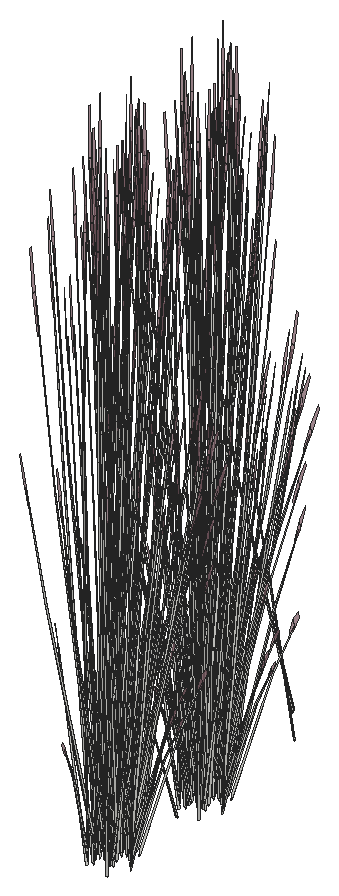
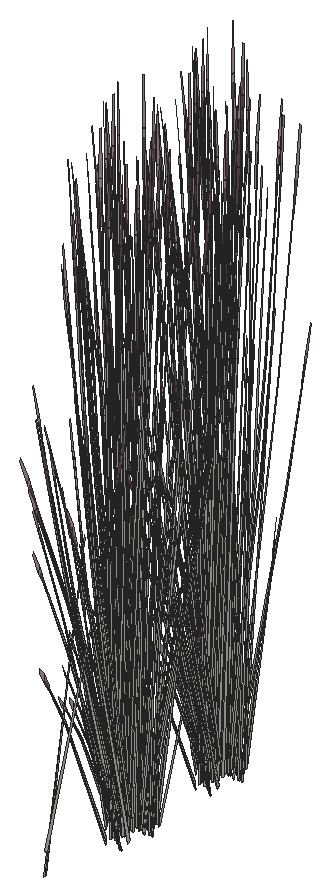
# SketchUp Ruby script. Lengths in inches.
U = 1.inch
M = Sketchup.active_model
def pt(a) = Geom::Point3d.new(a.map { |v| v * U })
def face(e, loops, mat)
  f = e.add_face(loops[0].map { |a| pt(a) })
  loops[1..].each { |l| e.add_face(l.map { |a| pt(a) }).erase! }
  f.material = f.back_material = mat if mat
  f
end
# faces: each face lists its corners as indices into pts; further lists are holes
def faces(e, pts, list, mat = nil) = list.each { |f| face(e, (f[0].is_a?(Array) ? f : [f]).map { |l| l.map { |i| pts[i] } }, mat) }
# xy, xz, yz: faces in a plane at the given z, y or x. An outline is a flat list of corners, or four numbers for a rectangle; further outlines are holes
def ring(l) = l.size == 4 ? [[l[0], l[1]], [l[2], l[1]], [l[2], l[3]], [l[0], l[3]]] : l.each_slice(2).to_a
def flat(e, list, mat, &to3) = list.each { |f| face(e, (f[0].is_a?(Array) ? f : [f]).map { |l| ring(l).map { |u, v| to3.(u, v) } }, mat) }
def xy(e, z, list, mat = nil) = flat(e, list, mat) { |x, y| [x, y, z] }
def xz(e, y, list, mat = nil) = flat(e, list, mat) { |x, z| [x, y, z] }
def yz(e, x, list, mat = nil) = flat(e, list, mat) { |y, z| [x, y, z] }
def lines(e, pts, list) = list.each { |a, b| e.add_line(pt(pts[a]), pt(pts[b])) }
# prism: a flat outline (further loops are holes) pulled along v
def prism(e, loops, v, mat = nil)
  f = face(e, loops, mat); d = Geom::Vector3d.new(v.map { |x| x * U })
  f.pushpull(f.normal.samedirection?(d) ? d.length : -d.length)
end
def box(e, o, s, mat = nil) = prism(e, [[o, [o[0] + s[0], o[1], o[2]], [o[0] + s[0], o[1] + s[1], o[2]], [o[0], o[1] + s[1], o[2]]]], [0, 0, s[2]], mat)
def at(x, y, z, deg = 0) = Geom::Transformation.translation(pt([x, y, z])) * Geom::Transformation.rotation(ORIGIN, Z_AXIS, deg.degrees)
def axes(o, x, y, z) = Geom::Transformation.new([*x, 0, *y, 0, *z, 0, *pt(o).to_a, 1])
def part(name) = M.definitions.add(name)
# library, detail: a bought-in or finely detailed component or shape, given as its bounding box
def library(name, o, s) = part(name).tap { |d| box(d.entities, o, s) }
def detail(e, o, s) = box(e.add_group.entities, o, s)
def put(e, d, t, mat = nil) = e.add_instance(d, t).tap { |i| i.material = mat if mat }
def group(e, t, mat = nil) = e.add_group.tap { |g| g.transformation = t; g.material = mat if mat }.entities
root = M.entities
M.materials.add("LightPink_Translucent").color = [144, 107, 117]
M.materials["LightPink_Translucent"].alpha = 0.75
c1 = part("blade")
p = [[2.15,0.21,22],[0,0.17,0],[0.09,0.45,0],[2.18,0.31,22],[2.29,0.31,22],[0.38,0.45,0],
  [2.48,0.24,33],[2.49,0.24,33],[2.48,0.22,33]]
faces(c1.entities,p,[[0,1,2,3],[4,5,2,3],[6,3,4,7],[8,0,3,6]])
c2 = part("seeds")
p = [[0.3,-0.1,1.38],[-0.01,-0.03,1.59],[-0.01,-0.03,0.03],[0.14,-0.07,-0.07],[0.29,-0.03,3],[0.15,0.01,3.11]]
faces(c2.entities,p,[[0,1,2,3],[1,0,4,5]],"LightPink_Translucent")
c3 = part("blade with seeds")
put(c3.entities,c1,at(0,0,0))
put(c3.entities,c2,axes([2.4,0.25,30.99],[1.5799,-0.05474,1.17369],[-0.12525,1.92788,0.29478],[-0.07173,-0.02425,1.56792]))
put(root,c3,axes([402.53,753.12,3.875],[-0.06572,0.16029,1.71376],[-0.27569,-0.33172,0.13857],[0.12437,-0.20675,0.73262]))
put(root,c3,axes([402.14,752.89,4.68],[-0.34695,-0.11691,-0.51099],[0.11892,-0.40083,-0.3958],[-0.03181,-0.16138,0.97773]))
put(root,c3,axes([402.35,751.88,2.77],[0.04528,0.27194,1.1486],[-0.25117,-0.15062,0.84392],[0.02703,-0.13924,0.25299]))
put(root,c3,axes([402.89,753.19,4.68],[-0.25266,-0.31335,-0.51099],[0.2669,-0.27442,-0.3958],[0.03844,-0.15921,0.97773]))
put(root,c3,axes([403.13,753.08,4.53],[0.23881,-0.24554,-0.35414],[0.22606,0.28036,0.4572],[0.0344,-0.14245,0.87481]))
put(root,c3,axes([401.49,754.39,2.1],[-0.14494,-0.47823,-0.69835],[0.41752,-0.17223,-0.18329],[-0.01602,-0.16194,1.54149]))
put(root,c3,axes([403.43,752.93,1.49],[-0.05283,-0.03674,1.76342],[-0.13569,-0.41045,-0.26939],[0.09154,-0.11138,0.30037]))
put(root,c3,axes([403.42,754.09,4.98],[0.18436,-0.36797,-0.71045],[0.32306,0.26151,0.08574],[0.11008,-0.13332,1.00501]))
put(root,c3,axes([401.43,753.01,2.375],[-0.22066,-0.46731,0],[0.36918,-0.26061,-0.51607],[0.08408,-0.05936,1.63711]))
put(root,c3,axes([403.41,753.91,4.68],[-0.09067,-0.42583,-0.51099],[0.34336,-0.07449,-0.3958],[0.0984,-0.11438,0.97773]))
put(root,c3,axes([401.92,752.45,2.13],[-0.2439,0.26754,-0.03893],[-0.22348,-0.29302,-0.17649],[-0.01573,-0.08303,0.58215]))
put(root,c3,axes([400.63,754.32,2.02],[0,-0.46636,-0.49651],[0.39487,0,0],[0,-0.10622,1.57504]))
put(root,c3,axes([401.73,752.94,2.02],[0.33032,-0.23318,-0.49651],[0.19744,0.41812,0],[0.07523,-0.05311,1.57504]))
put(root,c3,axes([403.69,753.75,2.59],[-0.12609,-0.01381,1.43002],[-0.12917,-0.37055,-0.30754],[0.1549,-0.10482,0.61141]))
put(root,c3,axes([402.12,753.9,2.06],[0.23773,-0.35053,-0.62353],[0.29532,0.31785,-0.16365],[0.09526,-0.08744,1.37633]))
put(root,c3,axes([403.84,753.07,2.77],[-0.11756,0.2374,1.1486],[-0.10105,-0.31895,0.84392],[0.09709,-0.07992,0.25299]))
put(root,c3,axes([403.67,753.96,4.53],[0.30722,-0.06665,-0.35414],[0.08112,0.381,0.4572],[0.08804,-0.10234,0.87481]))
put(root,c3,axes([401.71,754.51,2.21],[0.17124,-0.42022,-0.44739],[0.35581,0.20224,0.21531],[0,-0.09687,1.43643]))
put(root,c3,axes([401.86,754.3,2.67],[-0.04113,-0.53214,-0.29095],[0.42835,-0.03218,-0.50002],[0.07543,-0.07088,1.59708]))
put(root,c3,axes([400.8,754.33,2.03],[0.24637,-0.29097,-0.30978],[0.24637,0.29097,0.30978],[0,-0.09372,1.38974]))
put(root,c3,axes([401.67,754.86,2.67],[-0.39748,-0.22252,-0.29095],[0.19139,-0.46966,-0.50002],[-0.01249,-0.11531,1.59708]))
put(root,c3,axes([401.81,753.125,2.03],[0.32928,0.11539,-0.30978],[-0.08291,0.40636,0.30978],[0.06638,-0.04686,1.38974]))
put(root,c3,axes([401.92,754.72,2.43],[0.39767,0.22603,0.24065],[-0.19139,0.46966,0.50002],[0,-0.10827,1.60543]))
put(root,c3,axes([401.79,754.41,2.72],[-0.38326,0.02879,0.44739],[-0.03466,-0.47788,-0.21531],[0.06861,-0.04843,1.43643]))
put(root,c3,axes([400.8,754.75,2.48],[0,0.46636,0.49651],[-0.39487,0,0],[0,-0.10622,1.57504]))
put(root,c3,axes([403.57,754.86,4.68],[0.09562,-0.42421,-0.51099],[0.32782,0.1454,-0.3958],[0.13199,-0.0389,0.97773]))
put(root,c3,axes([403.06,753.13,2.375],[0.22066,-0.46731,0],[0.36918,0.26061,-0.51607],[0.08408,0.05936,1.63711]))
put(root,c3,axes([401.78,754.58,2.36],[0.15345,0.52148,0.45755],[-0.43845,0.18134,0.17955],[0.00536,-0.09582,1.58856]))
put(root,c3,axes([403.92,754.98,1.98],[-0.22732,0.05597,1.41583],[-0.03618,-0.44548,0.08104],[0.15921,-0.06743,0.80566]))
put(root,c3,axes([404.34,754.58,2.26],[-0.21881,-0.29821,-0.06488],[0.23965,-0.27324,-0.29416],[0.0679,-0.01924,0.97024]))
put(root,c3,axes([401.7,754.99,2.72],[-0.17124,0.42022,0.44739],[-0.35581,-0.20224,-0.21531],[0,-0.09687,1.43643]))
put(root,c3,axes([402.33,754.62,2.21],[0,-0.53961,0],[0.44133,0,0],[0,0,1.79456]))
put(root,c3,axes([402.87,753.375,2.48],[-0.33032,-0.23318,0.49651],[0.19744,-0.41812,0],[0.07523,0.05311,1.57504]))
put(root,c3,axes([403.51,755.01,4.98],[0.31014,-0.20596,-0.71045],[0.17284,0.42397,0.08574],[0.14985,-0.04816,1.00501]))
put(root,c3,axes([402.12,754.28,2.36],[-0.29264,0.42323,0.45755],[-0.34767,-0.3736,0.17955],[0.07055,-0.04224,1.58856]))
put(root,c3,axes([402.44,755.04,2.3],[-0.32829,-0.4014,-0.06131],[0.32849,-0.40164,0],[-0.01146,-0.01402,1.75571]))
put(root,c3,axes([401.61,753.59,2.47],[-0.10196,0.46348,0.17642],[-0.3731,-0.13116,0.35086],[0.06445,-0.00226,1.60407]))
put(root,c3,axes([401.46,753.96,1.59],[-0.3474,0.18671,1.28929],[-0.11057,-0.53572,0.50096],[0.21332,0.00891,1.46642]))
put(root,c3,axes([402.39,754.1,2.62],[0.06809,-0.4162,0.1448],[0.33266,0.07225,-0.41347],[0.06054,0.04274,1.26744]))
put(root,c3,axes([401.82,755.09,2.36],[0.44609,0.09826,0.45755],[-0.09078,0.55493,0.17955],[-0.06519,-0.05359,1.58856]))
put(root,c3,axes([404.17,754.6875,1.49],[-0.01845,-0.0708,1.76342],[0.12793,-0.41416,-0.26939],[0.12905,-0.00596,0.30037]))
put(root,c3,axes([402.25,754.21,2.72],[-0.21202,-0.39143,0.44739],[0.32115,-0.27564,-0.21531],[0.06861,0.04843,1.43643]))
put(root,c3,axes([401.58,755.98,2.47],[0.37926,-0.12378,0.17642],[0.09365,0.46065,0.35086],[-0.03382,-0.06712,1.60407]))
put(root,c3,axes([402.36,754.24,2.67],[0.35635,-0.30962,-0.29095],[0.23697,0.43749,-0.50002],[0.08792,0.04443,1.59708]))
put(root,c3,axes([403.78,755.05,4.53],[0.29332,0.1301,-0.35414],[-0.08555,0.37955,0.4572],[0.11809,-0.0348,0.87481]))
put(root,c3,axes([403.26,753.41,2.02],[0.33032,0.23318,-0.49651],[-0.19744,0.41812,0],[0.07523,0.05311,1.57504]))
put(root,c3,axes([402.63,754.74,2.21],[0.39487,0,0],[0,0.48281,0],[0,0,1.78407]))
put(root,c3,axes([402.74,753.61,2.47],[-0.37926,0.12378,0.17642],[-0.09365,-0.46065,0.35086],[0.03382,0.06712,1.60407]))
put(root,c3,axes([402.98,754.58,3.875],[-0.14639,0.01056,1.71376],[0.09712,-0.45778,0.13857],[0.20862,0.02831,0.73262]))
put(root,c3,axes([403.17,753.59,2.03],[0.08291,0.40636,-0.30978],[-0.32928,0.11539,0.30978],[0.06638,0.04686,1.38974]))
put(root,c3,axes([402.5,754.5,2.38],[-0.44609,-0.09826,0.49198],[0.09078,-0.55493,0.19306],[0.06519,0.05359,1.70813]))
put(root,c3,axes([402.15,755.87,2.2],[-0.11516,-0.40207,0],[0.32884,-0.1408,0],[0,0,1.54371]))
put(root,c3,axes([402.58,755.8125,2.18],[0.37054,-0.15823,-0.19198],[0.1302,0.45581,0.00008],[0.0409,-0.01749,1.73897]))
put(root,c3,axes([402.71,756,2.47],[0.10196,-0.46348,0.17642],[0.3731,0.13116,0.35086],[-0.06445,0.00226,1.60407]))
put(root,c3,axes([402.62,754.95,2.21],[0.24637,0.30123,0],[-0.24637,0.30123,0],[0,0,1.69266]))
put(root,c3,axes([403.29,754.82,2.47],[-0.2773,-0.3397,0.17642],[0.27945,-0.32949,0.35086],[-0.03063,0.06937,1.60407]))
put(root,c3,axes([402.78,754.31,2.06],[0.36714,0.07646,-0.62353],[-0.07747,0.47163,-0.16365],[0.10956,0.05715,1.37633]))
put(root,c3,axes([404.4,755.13,2.77],[-0.21807,0.07699,1.1486],[0.10265,-0.31819,0.84392],[0.11568,0.02177,0.25299]))
put(root,c3,axes([402.07,756.05,2.2],[-0.35581,-0.20937,0],[0.17124,-0.43505,0],[0,0,1.62707]))
put(root,c3,axes([402.62,754.6,2.72],[0.17124,-0.42022,0.44739],[0.35581,0.20224,-0.21531],[0,0.09687,1.43643]))
put(root,c3,axes([402.55,754.84,2.29],[0,0.53934,-0.05637],[-0.44133,0,0],[0,0.01695,1.79368]))
put(root,c3,axes([402.58,754.46,2.21],[0.21202,0.39143,-0.44739],[-0.32115,0.27564,0.21531],[0.06861,0.04843,1.43643]))
put(root,c3,axes([404.02,756.11,3.93],[-0.06755,-0.39203,-0.03492],[0.31928,-0.09013,-0.15832],[0.06667,0.02485,0.52218]))
put(root,c3,axes([403.52,754.83,2.48],[0,-0.46636,0.49651],[0.39487,0,0],[0,0.10622,1.57504]))
put(root,c3,axes([402.53,755.18,2.72],[0.38326,-0.02879,0.44739],[0.03466,0.47788,-0.21531],[-0.06861,0.04843,1.43643]))
put(root,c3,axes([402.77,754.69,2.62],[0.32884,-0.136,0.1448],[0.11516,0.38837,-0.41347],[0,0.08547,1.26744]))
put(root,c3,axes([403.99,755.64,2.59],[-0.085,-0.1147,1.43002],[0.1106,-0.37943,-0.30754],[0.17198,0.0514,0.61141]))
put(root,c3,axes([402.47,756.06,2.2],[0.35581,0.20937,0],[-0.17124,0.43505,0],[0,0,1.74954]))
put(root,c3,axes([402.61,756.52,2.19],[-0.21791,-0.46895,-0.05142],[0.36918,-0.26061,0.51607],[-0.09097,0.04465,1.6363]))
put(root,c3,axes([402.53,755.39,2.62],[0.26075,0.2802,0.1448],[-0.2175,0.31612,-0.41347],[-0.06054,0.04274,1.26744]))
put(root,c3,axes([403.21,755.87,4.98],[0.35281,0.01123,-0.71045],[-0.0237,0.47284,0.08574],[0.14947,0.0499,1.00501]))
put(root,c3,axes([402.8125,756.25,2.48],[0.33032,-0.23318,0.49651],[0.19744,0.41812,0],[-0.07523,0.05311,1.57504]))
put(root,c3,axes([402.34,755.88,2.29],[0.15345,0.53576,-0.06012],[-0.43845,0.18773,0],[0.00536,0.01871,1.72173]))
put(root,c3,axes([402.51,756.46,2.03],[-0.32928,-0.11539,-0.30978],[0.08291,-0.40636,0.30978],[-0.06638,0.04686,1.38974]))
put(root,c3,axes([403.78,754.91,2.375],[0.44133,0,0],[0,0.52122,-0.51607],[0,0.11871,1.63711]))
put(root,c3,axes([403.61,755.18,2.2],[-0.44111,-0.00373,-0.04976],[0,-0.52122,0.49943],[-0.01386,0.11865,1.58352]))
put(root,c3,axes([402.65,754.73,2.67],[0.39748,0.22252,-0.29095],[-0.19139,0.46966,-0.50002],[0.01249,0.11531,1.59708]))
put(root,c3,axes([403.42,756.07,4.53],[0.20082,0.29199,-0.35414],[-0.2293,0.2764,0.4572],[0.1165,0.04206,0.87481]))
put(root,c3,axes([403.52,755.25,2.03],[-0.24637,0.29097,-0.30978],[-0.24637,-0.29097,0.30978],[0,0.09372,1.38974]))
put(root,c3,axes([402.46,755.28,2.67],[0.04113,0.53214,-0.29095],[-0.42835,0.03218,-0.50002],[-0.07543,0.07088,1.59708]))
put(root,c3,axes([402.61,755.07,2.21],[-0.17124,0.42022,-0.44739],[-0.35581,-0.20224,0.21531],[0,0.09687,1.43643]))
put(root,c3,axes([402.62,756.28,2.33],[0.44186,0.15158,0.30756],[-0.11054,0.54181,-0.36492],[-0.07313,0.06781,1.64885]))
put(root,c3,axes([402.59,756.65,2.02],[-0.33032,0.23318,-0.49651],[-0.19744,-0.41812,0],[-0.07523,0.05311,1.57504]))
put(root,c3,axes([403.6875,755.26,2.02],[0,0.46636,-0.49651],[-0.39487,0,0],[0,0.10622,1.57504]))
put(root,c3,axes([402.7,755.32,3.875],[-0.1311,-0.08035,1.71376],[0.27131,-0.33708,0.13857],[0.16909,0.15206,0.73262]))
put(root,c3,axes([403.18,756.23,2.77],[-0.19872,-0.13409,1.1486],[0.2566,-0.13625,0.84392],[0.06921,0.11541,0.25299]))
put(root,c3,axes([402.89,756.57,2.375],[0.22066,0.46731,0],[-0.36918,0.26061,-0.51607],[-0.08408,0.05936,1.63711]))
put(root,c3,axes([403.24,756.73,1.49],[0.02571,-0.06733,1.76342],[0.32373,-0.19829,-0.26939],[0.09815,0.10263,0.30037]))
put(root,c3,axes([402.7,754.72,2.84],[-0.00964,-0.43909,1.41272],[0.43635,0.11382,0.59816],[-0.1032,0.24027,1.3335]))
put(root,c3,axes([402.8125,755.2,2.09],[0.12941,0.42699,-0.69212],[-0.37279,0.15378,-0.18165],[0.0143,0.14459,1.52773]))
put(root,c3,axes([402.74,756.42,4.68],[0.34827,-0.11086,-0.51099],[0.06092,0.41983,-0.3958],[0.09354,0.12031,0.97773]))
put(root,c3,axes([403.22,756.84,2.67],[-0.22633,-0.01463,1.0506],[0.14947,-0.31064,0.58006],[0.08941,0.11036,0.8241]))
put(root,c3,axes([402.48,756.09,2.59],[0.00623,-0.15459,1.43002],[0.29764,-0.17268,-0.30754],[0.09188,0.18503,0.61141]))
put(root,c3,axes([401.73,756.72,1.49],[0.05712,-0.02538,1.76342],[0.34359,0.13968,-0.26939],[0.01005,0.15742,0.30037]))
put(root,c3,axes([401.21,756.31,5],[0.25266,0.31335,-0.5672],[-0.2669,0.27442,-0.43934],[-0.03844,0.15921,1.08528]))
put(root,c3,axes([400.9375,756.78,2.82],[0.32063,-0.08258,0.06507],[0.07371,0.33271,-0.86304],[-0.02033,0.16842,0.7736]))
put(root,c3,axes([401.96,756.61,4.68],[0.34695,0.11691,-0.51099],[-0.11892,0.40083,-0.3958],[0.03181,0.16138,0.97773]))
put(root,c3,axes([402.16,755.78,3.875],[-0.08068,-0.14973,1.71376],[0.3728,-0.12606,0.13857],[0.08426,0.23506,0.73262]))
put(root,c3,axes([402.72,763.4375,2.59],[-0.10032,0.0944,1.43002],[-0.30046,-0.16522,-0.30754],[0.05569,-0.20547,0.61141]))
put(root,c3,axes([402.27,763.77,4.98],[-0.16845,-0.3792,-0.71045],[0.34676,-0.21133,0.08574],[-0.03939,-0.18322,1.00501]))
put(root,c3,axes([401.8,756.86,4.53],[-0.1064,0.35863,-0.35414],[-0.31043,-0.1046,0.4572],[0.02846,0.14439,0.87481]))
put(root,c3,axes([401.98,762.93,1.49],[-0.0592,0.0168,1.76342],[-0.32738,-0.18913,-0.26939],[0.00549,-0.15776,0.30037]))
put(root,c3,axes([402.97,764.14,4.98],[0.00918,-0.43138,-0.71045],[0.38672,0.02897,0.08574],[0.04081,-0.18275,1.00501]))
put(root,c3,axes([401.5,755.86,3.875],[-0.00864,-0.17899,1.71376],[0.37441,0.11874,0.13857],[-0.02316,0.25508,0.73262]))
put(root,c3,axes([402.3,763.45,4.53],[0.1064,-0.35863,-0.35414],[0.31043,0.1046,0.4572],[-0.02846,-0.14439,0.87481]))
put(root,c3,axes([402.53,763.92,3.875],[-0.06572,0.16029,1.71376],[-0.27569,-0.33172,0.13857],[0.12437,-0.20675,0.73262]))
put(root,c3,axes([401.84,756.54,4.98],[0.16845,0.3792,-0.71045],[-0.34676,0.21133,0.08574],[0.03939,0.18322,1.00501]))
put(root,c3,axes([402.14,763.69,4.68],[-0.34695,-0.11691,-0.51099],[0.11892,-0.40083,-0.3958],[-0.03181,-0.16138,0.97773]))
put(root,c3,axes([402.35,762.6875,2.77],[0.04528,0.27194,1.1486],[-0.25117,-0.15062,0.84392],[0.02703,-0.13924,0.25299]))
put(root,c3,axes([402.89,763.99,4.68],[-0.25266,-0.31335,-0.51099],[0.2669,-0.27442,-0.3958],[0.03844,-0.15921,0.97773]))
put(root,c3,axes([403.13,763.88,4.53],[0.23881,-0.24554,-0.35414],[0.22606,0.28036,0.4572],[0.0344,-0.14245,0.87481]))
put(root,c3,axes([401.49,765.19,2.1],[-0.14494,-0.47823,-0.69835],[0.41752,-0.17223,-0.18329],[-0.01602,-0.16194,1.54149]))
put(root,c3,axes([403.43,763.73,1.49],[-0.05283,-0.03674,1.76342],[-0.13569,-0.41045,-0.26939],[0.09154,-0.11138,0.30037]))
put(root,c3,axes([403.42,764.89,4.98],[0.18436,-0.36797,-0.71045],[0.32306,0.26151,0.08574],[0.11008,-0.13332,1.00501]))
put(root,c3,axes([401.43,763.82,2.375],[-0.22066,-0.46731,0],[0.36918,-0.26061,-0.51607],[0.08408,-0.05936,1.63711]))
put(root,c3,axes([403.41,764.72,4.68],[-0.09067,-0.42583,-0.51099],[0.34336,-0.07449,-0.3958],[0.0984,-0.11438,0.97773]))
put(root,c3,axes([401.92,763.25,2.13],[-0.2439,0.26754,-0.03893],[-0.22348,-0.29302,-0.17649],[-0.01573,-0.08303,0.58215]))
put(root,c3,axes([400.63,765.125,2.02],[0,-0.46636,-0.49651],[0.39487,0,0],[0,-0.10622,1.57504]))
put(root,c3,axes([401.73,763.74,2.02],[0.33032,-0.23318,-0.49651],[0.19744,0.41812,0],[0.07523,-0.05311,1.57504]))
put(root,c3,axes([403.69,764.55,2.59],[-0.12609,-0.01381,1.43002],[-0.12917,-0.37055,-0.30754],[0.1549,-0.10482,0.61141]))
put(root,c3,axes([402.12,764.7,2.06],[0.23773,-0.35053,-0.62353],[0.29532,0.31785,-0.16365],[0.09526,-0.08744,1.37633]))
put(root,c3,axes([403.84,763.87,2.77],[-0.11756,0.2374,1.1486],[-0.10105,-0.31895,0.84392],[0.09709,-0.07992,0.25299]))
put(root,c3,axes([403.67,764.76,4.53],[0.30722,-0.06665,-0.35414],[0.08112,0.381,0.4572],[0.08804,-0.10234,0.87481]))
put(root,c3,axes([401.71,765.32,2.21],[0.17124,-0.42022,-0.44739],[0.35581,0.20224,0.21531],[0,-0.09687,1.43643]))
put(root,c3,axes([401.86,765.11,2.67],[-0.04113,-0.53214,-0.29095],[0.42835,-0.03218,-0.50002],[0.07543,-0.07088,1.59708]))
put(root,c3,axes([400.8,765.13,2.03],[0.24637,-0.29097,-0.30978],[0.24637,0.29097,0.30978],[0,-0.09372,1.38974]))
put(root,c3,axes([401.67,765.66,2.67],[-0.39748,-0.22252,-0.29095],[0.19139,-0.46966,-0.50002],[-0.01249,-0.11531,1.59708]))
put(root,c3,axes([401.81,763.93,2.03],[0.32928,0.11539,-0.30978],[-0.08291,0.40636,0.30978],[0.06638,-0.04686,1.38974]))
put(root,c3,axes([401.92,765.52,2.43],[0.39767,0.22603,0.24065],[-0.19139,0.46966,0.50002],[0,-0.10827,1.60543]))
put(root,c3,axes([401.79,765.21,2.72],[-0.38326,0.02879,0.44739],[-0.03466,-0.47788,-0.21531],[0.06861,-0.04843,1.43643]))
put(root,c3,axes([400.8,765.56,2.48],[0,0.46636,0.49651],[-0.39487,0,0],[0,-0.10622,1.57504]))
put(root,c3,axes([403.57,765.66,4.68],[0.09562,-0.42421,-0.51099],[0.32782,0.1454,-0.3958],[0.13199,-0.0389,0.97773]))
put(root,c3,axes([403.06,763.93,2.375],[0.22066,-0.46731,0],[0.36918,0.26061,-0.51607],[0.08408,0.05936,1.63711]))
put(root,c3,axes([401.78,765.38,2.36],[0.15345,0.52148,0.45755],[-0.43845,0.18134,0.17955],[0.00536,-0.09582,1.58856]))
put(root,c3,axes([403.92,765.78,1.98],[-0.22732,0.05597,1.41583],[-0.03618,-0.44548,0.08104],[0.15921,-0.06743,0.80566]))
put(root,c3,axes([404.34,765.39,2.26],[-0.21881,-0.29821,-0.06488],[0.23965,-0.27324,-0.29416],[0.0679,-0.01924,0.97024]))
put(root,c3,axes([401.7,765.79,2.72],[-0.17124,0.42022,0.44739],[-0.35581,-0.20224,-0.21531],[0,-0.09687,1.43643]))
put(root,c3,axes([402.33,765.43,2.21],[0,-0.53961,0],[0.44133,0,0],[0,0,1.79456]))
put(root,c3,axes([402.87,764.18,2.48],[-0.33032,-0.23318,0.49651],[0.19744,-0.41812,0],[0.07523,0.05311,1.57504]))
put(root,c3,axes([403.51,765.82,4.98],[0.31014,-0.20596,-0.71045],[0.17284,0.42397,0.08574],[0.14985,-0.04816,1.00501]))
put(root,c3,axes([402.12,765.09,2.36],[-0.29264,0.42323,0.45755],[-0.34767,-0.3736,0.17955],[0.07055,-0.04224,1.58856]))
put(root,c3,axes([402.44,765.84,2.3],[-0.32829,-0.4014,-0.06131],[0.32849,-0.40164,0],[-0.01146,-0.01402,1.75571]))
put(root,c3,axes([401.61,764.39,2.47],[-0.10196,0.46348,0.17642],[-0.3731,-0.13116,0.35086],[0.06445,-0.00226,1.60407]))
put(root,c3,axes([401.46,764.76,1.59],[-0.3474,0.18671,1.28929],[-0.11057,-0.53572,0.50096],[0.21332,0.00891,1.46642]))
put(root,c3,axes([402.39,764.9,2.62],[0.06809,-0.4162,0.1448],[0.33266,0.07225,-0.41347],[0.06054,0.04274,1.26744]))
put(root,c3,axes([401.82,765.89,2.36],[0.44609,0.09826,0.45755],[-0.09078,0.55493,0.17955],[-0.06519,-0.05359,1.58856]))
put(root,c3,axes([404.17,765.49,1.49],[-0.01845,-0.0708,1.76342],[0.12793,-0.41416,-0.26939],[0.12905,-0.00596,0.30037]))
put(root,c3,axes([402.25,765.01,2.72],[-0.21202,-0.39143,0.44739],[0.32115,-0.27564,-0.21531],[0.06861,0.04843,1.43643]))
put(root,c3,axes([401.58,766.78,2.47],[0.37926,-0.12378,0.17642],[0.09365,0.46065,0.35086],[-0.03382,-0.06712,1.60407]))
put(root,c3,axes([402.36,765.04,2.67],[0.35635,-0.30962,-0.29095],[0.23697,0.43749,-0.50002],[0.08792,0.04443,1.59708]))
put(root,c3,axes([403.78,765.86,4.53],[0.29332,0.1301,-0.35414],[-0.08555,0.37955,0.4572],[0.11809,-0.0348,0.87481]))
put(root,c3,axes([403.26,764.22,2.02],[0.33032,0.23318,-0.49651],[-0.19744,0.41812,0],[0.07523,0.05311,1.57504]))
put(root,c3,axes([402.63,765.55,2.21],[0.39487,0,0],[0,0.48281,0],[0,0,1.78407]))
put(root,c3,axes([402.74,764.41,2.47],[-0.37926,0.12378,0.17642],[-0.09365,-0.46065,0.35086],[0.03382,0.06712,1.60407]))
put(root,c3,axes([402.98,765.39,3.875],[-0.14639,0.01056,1.71376],[0.09712,-0.45778,0.13857],[0.20862,0.02831,0.73262]))
put(root,c3,axes([403.17,764.39,2.03],[0.08291,0.40636,-0.30978],[-0.32928,0.11539,0.30978],[0.06638,0.04686,1.38974]))
put(root,c3,axes([402.5,765.3,2.38],[-0.44609,-0.09826,0.49198],[0.09078,-0.55493,0.19306],[0.06519,0.05359,1.70813]))
put(root,c3,axes([402.15,766.67,2.2],[-0.11516,-0.40207,0],[0.32884,-0.1408,0],[0,0,1.54371]))
put(root,c3,axes([402.58,766.61,2.18],[0.37054,-0.15823,-0.19198],[0.1302,0.45581,0.00008],[0.0409,-0.01749,1.73897]))
put(root,c3,axes([402.71,766.8,2.47],[0.10196,-0.46348,0.17642],[0.3731,0.13116,0.35086],[-0.06445,0.00226,1.60407]))
put(root,c3,axes([402.62,765.75,2.21],[0.24637,0.30123,0],[-0.24637,0.30123,0],[0,0,1.69266]))
put(root,c3,axes([403.29,765.62,2.47],[-0.2773,-0.3397,0.17642],[0.27945,-0.32949,0.35086],[-0.03063,0.06937,1.60407]))
put(root,c3,axes([402.78,765.11,2.06],[0.36714,0.07646,-0.62353],[-0.07747,0.47163,-0.16365],[0.10956,0.05715,1.37633]))
put(root,c3,axes([404.4,765.93,2.77],[-0.21807,0.07699,1.1486],[0.10265,-0.31819,0.84392],[0.11568,0.02177,0.25299]))
put(root,c3,axes([402.07,766.85,2.2],[-0.35581,-0.20937,0],[0.17124,-0.43505,0],[0,0,1.62707]))
put(root,c3,axes([402.62,765.4,2.72],[0.17124,-0.42022,0.44739],[0.35581,0.20224,-0.21531],[0,0.09687,1.43643]))
put(root,c3,axes([402.55,765.64,2.29],[0,0.53934,-0.05637],[-0.44133,0,0],[0,0.01695,1.79368]))
put(root,c3,axes([402.58,765.26,2.21],[0.21202,0.39143,-0.44739],[-0.32115,0.27564,0.21531],[0.06861,0.04843,1.43643]))
put(root,c3,axes([404.02,766.91,3.93],[-0.06755,-0.39203,-0.03492],[0.31928,-0.09013,-0.15832],[0.06667,0.02485,0.52218]))
put(root,c3,axes([403.52,765.63,2.48],[0,-0.46636,0.49651],[0.39487,0,0],[0,0.10622,1.57504]))
put(root,c3,axes([402.53,765.98,2.72],[0.38326,-0.02879,0.44739],[0.03466,0.47788,-0.21531],[-0.06861,0.04843,1.43643]))
put(root,c3,axes([402.77,765.5,2.62],[0.32884,-0.136,0.1448],[0.11516,0.38837,-0.41347],[0,0.08547,1.26744]))
put(root,c3,axes([403.99,766.44,2.59],[-0.085,-0.1147,1.43002],[0.1106,-0.37943,-0.30754],[0.17198,0.0514,0.61141]))
put(root,c3,axes([402.47,766.86,2.2],[0.35581,0.20937,0],[-0.17124,0.43505,0],[0,0,1.74954]))
put(root,c3,axes([402.61,767.32,2.19],[-0.21791,-0.46895,-0.05142],[0.36918,-0.26061,0.51607],[-0.09097,0.04465,1.6363]))
put(root,c3,axes([402.53,766.1875,2.62],[0.26075,0.2802,0.1448],[-0.2175,0.31612,-0.41347],[-0.06054,0.04274,1.26744]))
put(root,c3,axes([403.21,766.67,4.98],[0.35281,0.01123,-0.71045],[-0.0237,0.47284,0.08574],[0.14947,0.0499,1.00501]))
put(root,c3,axes([402.8125,767.05,2.48],[0.33032,-0.23318,0.49651],[0.19744,0.41812,0],[-0.07523,0.05311,1.57504]))
put(root,c3,axes([402.34,766.68,2.29],[0.15345,0.53576,-0.06012],[-0.43845,0.18773,0],[0.00536,0.01871,1.72173]))
put(root,c3,axes([402.51,767.26,2.03],[-0.32928,-0.11539,-0.30978],[0.08291,-0.40636,0.30978],[-0.06638,0.04686,1.38974]))
put(root,c3,axes([403.78,765.71,2.375],[0.44133,0,0],[0,0.52122,-0.51607],[0,0.11871,1.63711]))
put(root,c3,axes([403.61,765.98,2.2],[-0.44111,-0.00373,-0.04976],[0,-0.52122,0.49943],[-0.01386,0.11865,1.58352]))
put(root,c3,axes([402.65,765.53,2.67],[0.39748,0.22252,-0.29095],[-0.19139,0.46966,-0.50002],[0.01249,0.11531,1.59708]))
put(root,c3,axes([403.42,766.87,4.53],[0.20082,0.29199,-0.35414],[-0.2293,0.2764,0.4572],[0.1165,0.04206,0.87481]))
put(root,c3,axes([403.52,766.06,2.03],[-0.24637,0.29097,-0.30978],[-0.24637,-0.29097,0.30978],[0,0.09372,1.38974]))
put(root,c3,axes([402.46,766.09,2.67],[0.04113,0.53214,-0.29095],[-0.42835,0.03218,-0.50002],[-0.07543,0.07088,1.59708]))
put(root,c3,axes([402.61,765.88,2.21],[-0.17124,0.42022,-0.44739],[-0.35581,-0.20224,0.21531],[0,0.09687,1.43643]))
put(root,c3,axes([402.62,767.08,2.33],[0.44186,0.15158,0.30756],[-0.11054,0.54181,-0.36492],[-0.07313,0.06781,1.64885]))
put(root,c3,axes([402.59,767.45,2.02],[-0.33032,0.23318,-0.49651],[-0.19744,-0.41812,0],[-0.07523,0.05311,1.57504]))
put(root,c3,axes([403.6875,766.07,2.02],[0,0.46636,-0.49651],[-0.39487,0,0],[0,0.10622,1.57504]))
put(root,c3,axes([402.7,766.12,3.875],[-0.1311,-0.08035,1.71376],[0.27131,-0.33708,0.13857],[0.16909,0.15206,0.73262]))
put(root,c3,axes([403.18,767.04,2.77],[-0.19872,-0.13409,1.1486],[0.2566,-0.13625,0.84392],[0.06921,0.11541,0.25299]))
put(root,c3,axes([402.89,767.375,2.375],[0.22066,0.46731,0],[-0.36918,0.26061,-0.51607],[-0.08408,0.05936,1.63711]))
put(root,c3,axes([403.24,767.53,1.49],[0.02571,-0.06733,1.76342],[0.32373,-0.19829,-0.26939],[0.09815,0.10263,0.30037]))
put(root,c3,axes([402.7,765.53,2.84],[-0.00964,-0.43909,1.41272],[0.43635,0.11382,0.59816],[-0.1032,0.24027,1.3335]))
put(root,c3,axes([402.8125,766,2.09],[0.12941,0.42699,-0.69212],[-0.37279,0.15378,-0.18165],[0.0143,0.14459,1.52773]))
put(root,c3,axes([402.74,767.22,4.68],[0.34827,-0.11086,-0.51099],[0.06092,0.41983,-0.3958],[0.09354,0.12031,0.97773]))
put(root,c3,axes([403.22,767.65,2.67],[-0.22633,-0.01463,1.0506],[0.14947,-0.31064,0.58006],[0.08941,0.11036,0.8241]))
put(root,c3,axes([402.48,766.89,2.59],[0.00623,-0.15459,1.43002],[0.29764,-0.17268,-0.30754],[0.09188,0.18503,0.61141]))
put(root,c3,axes([401.73,767.52,1.49],[0.05712,-0.02538,1.76342],[0.34359,0.13968,-0.26939],[0.01005,0.15742,0.30037]))
put(root,c3,axes([401.21,767.11,5],[0.25266,0.31335,-0.5672],[-0.2669,0.27442,-0.43934],[-0.03844,0.15921,1.08528]))
put(root,c3,axes([400.9375,767.58,2.82],[0.32063,-0.08258,0.06507],[0.07371,0.33271,-0.86304],[-0.02033,0.16842,0.7736]))
put(root,c3,axes([401.96,767.41,4.68],[0.34695,0.11691,-0.51099],[-0.11892,0.40083,-0.3958],[0.03181,0.16138,0.97773]))
put(root,c3,axes([402.16,766.59,3.875],[-0.08068,-0.14973,1.71376],[0.3728,-0.12606,0.13857],[0.08426,0.23506,0.73262]))
put(root,c3,axes([401.8,767.66,4.53],[-0.1064,0.35863,-0.35414],[-0.31043,-0.1046,0.4572],[0.02846,0.14439,0.87481]))
put(root,c3,axes([401.5,766.66,3.875],[-0.00864,-0.17899,1.71376],[0.37441,0.11874,0.13857],[-0.02316,0.25508,0.73262]))
put(root,c3,axes([401.84,767.34,4.98],[0.16845,0.3792,-0.71045],[-0.34676,0.21133,0.08574],[0.03939,0.18322,1.00501]))
put(root,c3,axes([402.72,775.82,2.59],[-0.10032,0.0944,1.43002],[-0.30046,-0.16522,-0.30754],[0.05569,-0.20547,0.61141]))
put(root,c3,axes([402.27,776.14,4.98],[-0.16845,-0.3792,-0.71045],[0.34676,-0.21133,0.08574],[-0.03939,-0.18322,1.00501]))
